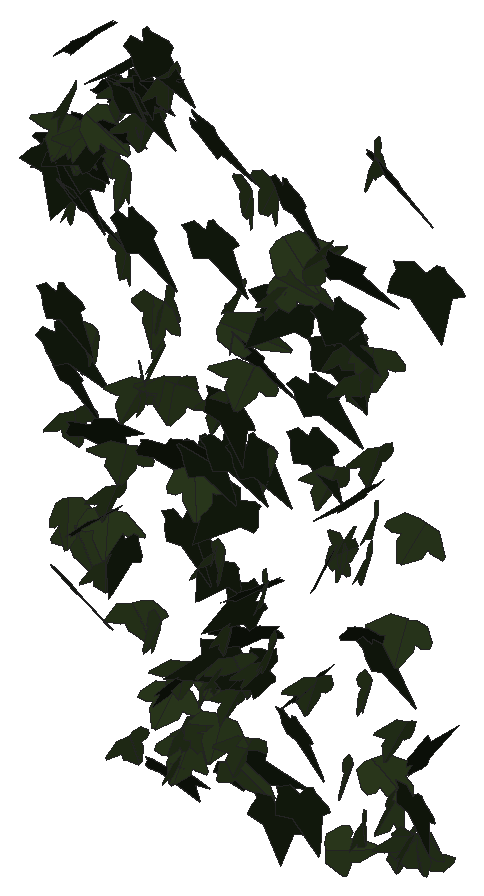
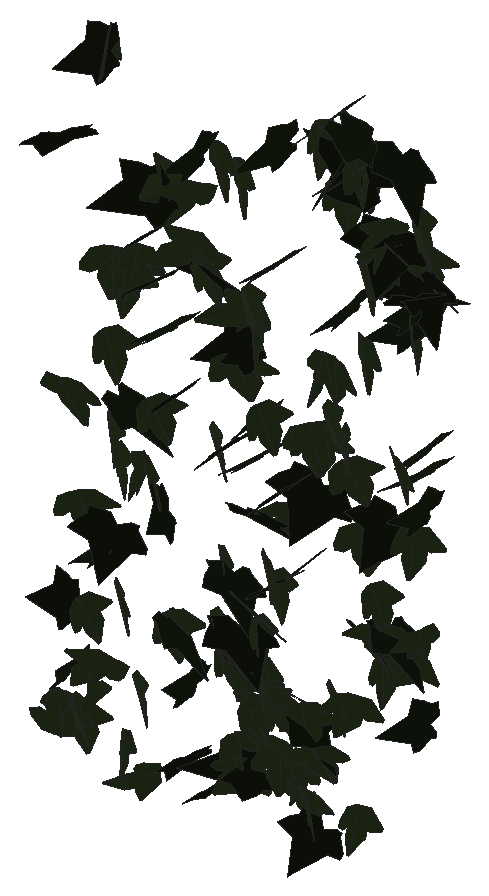
# SketchUp Ruby script. Lengths in inches.
U = 1.inch
M = Sketchup.active_model
def pt(a) = Geom::Point3d.new(a.map { |v| v * U })
def face(e, loops, mat)
  f = e.add_face(loops[0].map { |a| pt(a) })
  loops[1..].each { |l| e.add_face(l.map { |a| pt(a) }).erase! }
  f.material = f.back_material = mat if mat
  f
end
# faces: each face lists its corners as indices into pts; further lists are holes
def faces(e, pts, list, mat = nil) = list.each { |f| face(e, (f[0].is_a?(Array) ? f : [f]).map { |l| l.map { |i| pts[i] } }, mat) }
# xy, xz, yz: faces in a plane at the given z, y or x. An outline is a flat list of corners, or four numbers for a rectangle; further outlines are holes
def ring(l) = l.size == 4 ? [[l[0], l[1]], [l[2], l[1]], [l[2], l[3]], [l[0], l[3]]] : l.each_slice(2).to_a
def flat(e, list, mat, &to3) = list.each { |f| face(e, (f[0].is_a?(Array) ? f : [f]).map { |l| ring(l).map { |u, v| to3.(u, v) } }, mat) }
def xy(e, z, list, mat = nil) = flat(e, list, mat) { |x, y| [x, y, z] }
def xz(e, y, list, mat = nil) = flat(e, list, mat) { |x, z| [x, y, z] }
def yz(e, x, list, mat = nil) = flat(e, list, mat) { |y, z| [x, y, z] }
def lines(e, pts, list) = list.each { |a, b| e.add_line(pt(pts[a]), pt(pts[b])) }
# prism: a flat outline (further loops are holes) pulled along v
def prism(e, loops, v, mat = nil)
  f = face(e, loops, mat); d = Geom::Vector3d.new(v.map { |x| x * U })
  f.pushpull(f.normal.samedirection?(d) ? d.length : -d.length)
end
def box(e, o, s, mat = nil) = prism(e, [[o, [o[0] + s[0], o[1], o[2]], [o[0] + s[0], o[1] + s[1], o[2]], [o[0], o[1] + s[1], o[2]]]], [0, 0, s[2]], mat)
def at(x, y, z, deg = 0) = Geom::Transformation.translation(pt([x, y, z])) * Geom::Transformation.rotation(ORIGIN, Z_AXIS, deg.degrees)
def axes(o, x, y, z) = Geom::Transformation.new([*x, 0, *y, 0, *z, 0, *pt(o).to_a, 1])
def part(name) = M.definitions.add(name)
# library, detail: a bought-in or finely detailed component or shape, given as its bounding box
def library(name, o, s) = part(name).tap { |d| box(d.entities, o, s) }
def detail(e, o, s) = box(e.add_group.entities, o, s)
def put(e, d, t, mat = nil) = e.add_instance(d, t).tap { |i| i.material = mat if mat }
def group(e, t, mat = nil) = e.add_group.tap { |g| g.transformation = t; g.material = mat if mat }.entities
root = M.entities
M.materials.add("1026 AP 7946 SUNNY SIDE UP").color = [254, 231, 186]
M.materials.add("efeu1").color = [18, 25, 13]
M.materials.add("efeu2").color = [43, 57, 29]
c1 = part("ivyleaf_9")
p = [[1.54,2.16,1.25],[1.36,2.04,1.19],[-0.21,0.99,0.68],[-0.71,1.11,0.82],[-0.85,0.86,0.67],[-0.8,0.17,0.21],
  [-0.9,-0.01,0.1],[-0.67,-0.16,-0.02],[-0.08,-0.08,-0.05],[-0.03,-0.6,-0.4],[0.65,-0.88,-0.66],[0.83,-0.6,-0.49],
  [1.29,-0.42,-0.43],[1.8125,-0.07,-0.26],[1.21,0.44,0.15]]
faces(c1.entities,p,[[0,1,2,3,4,5,6,7,8,9,10,11,12,13,14]],"efeu1")
c2 = part("ivyleaf_10")
p = [[0,0.5,-0.03],[-0.0625,2.02,-0.43],[-0.19,2.01,-0.46],[-0.54,1.05,-0.29],[-0.52,0.625,-0.18],[-0.83,0.76,-0.28],
  [-1.16,0.64,-0.33],[-1.15,0.33,-0.24],[-0.77,-0.39,0.02],[-0.3,-0.51,0.16],[0.04,-0.48,0.23],[-0.02,2.01,-0.4375],
  [-0.06,2.01,-0.43],[0.04,-0.49,0.23],[0.67,-0.49,0.14],[1.38,0.36,-0.2],[1.375,0.51,-0.24],[0.81,0.65,-0.19],
  [0.62,0.59,-0.15],[0.6,1.09,-0.28],[0.5,1.23,-0.31]]
faces(c2.entities,p,[[0,1,2,3,4,5,6,7,8,9,10],[11,12,0,13,14,15,16,17,18,19,20]],"efeu2")
put(root,c1,axes([106.4,212.93,277.375],[0.2839,0.0766,-0.23567],[-0.3054,-0.12423,-0.20113],[-0.22609,0.264,-0.02425]),"1026 AP 7946 SUNNY SIDE UP")
put(root,c1,axes([106.09,213.01,274.86],[0.17298,-0.2627,-0.04258],[-0.00188,0.04263,-0.29273],[0.41779,0.10896,0.01631]),"1026 AP 7946 SUNNY SIDE UP")
put(root,c2,axes([106.47,212.88,277.74],[-0.41886,-0.09591,0.10877],[-0.09337,-0.12993,-0.27529],[0.20462,-0.25562,0.09702]),"1026 AP 7946 SUNNY SIDE UP")
put(root,c1,axes([106.36,212.98,277.13],[-0.301,-0.22812,-0.01885],[0.0526,-0.00599,-0.30532],[0.35582,-0.19209,0.02919]),"1026 AP 7946 SUNNY SIDE UP")
put(root,c2,axes([106.41,212.86,278.23],[0.10324,-0.30101,-0.0027],[0.009,0.00218,-0.31732],[0.47323,0.06563,0.00662]),"1026 AP 7946 SUNNY SIDE UP")
put(root,c2,axes([106.43,212.95,276.625],[0.10557,-0.27977,-0.07671],[0.01457,0.07686,-0.29473],[0.45436,0.06254,0.02728]),"1026 AP 7946 SUNNY SIDE UP")
put(root,c1,axes([106.18,212.98,273.81],[0.24349,-0.23616,0.02494],[0.02197,-0.02139,-0.29105],[0.37285,0.15548,0.00086]),"1026 AP 7946 SUNNY SIDE UP")
put(root,c1,axes([106.1875,212.96,270.41],[0.33257,-0.16333,0.03171],[0.0441,-0.01556,-0.27534],[0.25787,0.2133,0.00618]),"1026 AP 7946 SUNNY SIDE UP")
put(root,c2,axes([106.46,212.79,271.65],[0.13349,0.26405,-0.0414],[-0.0605,-0.03121,-0.28458],[-0.41595,0.08928,0.02811]),"1026 AP 7946 SUNNY SIDE UP")
put(root,c1,axes([106.25,212.8,274.36],[0.22668,-0.22817,-0.09832],[0.03052,0.11916,-0.26622],[0.38691,0.12427,0.0786]),"1026 AP 7946 SUNNY SIDE UP")
put(root,c1,axes([106.64,212.94,279.24],[-0.00906,0.30791,-0.01019],[0.00025,-0.01164,-0.31733],[-0.4845,-0.00576,0.00003]),"1026 AP 7946 SUNNY SIDE UP")
put(root,c1,axes([106.78,212.89,277.62],[-0.42856,0.13326,-0.00751],[-0.00462,-0.02428,-0.31178],[-0.20987,-0.27159,0.02221]),"1026 AP 7946 SUNNY SIDE UP")
put(root,c1,axes([106.3,212.99,276.97],[0.21519,-0.26095,0.03754],[0.01848,-0.03665,-0.3037],[0.41422,0.1372,-0.00595]),"1026 AP 7946 SUNNY SIDE UP")
put(root,c2,axes([106.56,212.79,273.18],[-0.18449,-0.25198,-0.06214],[0.05598,0.04833,-0.28582],[0.40303,-0.12206,0.01125]),"1026 AP 7946 SUNNY SIDE UP")
put(root,c1,axes([106.37,212.95,276.6875],[0.3311,-0.20967,0.01469],[0.04497,0.0069,-0.305],[0.3275,0.21102,0.02702]),"1026 AP 7946 SUNNY SIDE UP")
put(root,c2,axes([106.75,212.9375,277.65],[-0.2452,-0.23978,0.09506],[-0.01978,-0.10224,-0.29192],[0.40428,-0.15044,0.04337]),"1026 AP 7946 SUNNY SIDE UP")
put(root,c2,axes([106.62,212.85,271.26],[-0.41291,-0.03751,-0.08835],[0.14606,-0.07797,-0.25898],[0.01547,-0.26495,0.087]),"1026 AP 7946 SUNNY SIDE UP")
put(root,c2,axes([106.6875,212.99,274.39],[0.29951,-0.21338,0.00264],[0.02536,0.00935,-0.29401],[0.33462,0.19028,0.01992]),"1026 AP 7946 SUNNY SIDE UP")
put(root,c1,axes([106.91,212.84,271.62],[-0.09208,0.26235,-0.08078],[-0.00605,-0.08248,-0.27658],[-0.43119,-0.05487,0.02113]),"1026 AP 7946 SUNNY SIDE UP")
put(root,c1,axes([106.84,212.92,277.91],[0.38313,0.13865,-0.12038],[-0.17923,-0.03679,-0.28809],[-0.22276,0.26806,0.02475]),"1026 AP 7946 SUNNY SIDE UP")
put(root,c2,axes([106.78,212.91,277.55],[0.23921,0.21136,0.16111],[0.01306,0.17544,-0.25352],[-0.4121,0.12825,0.08548]),"1026 AP 7946 SUNNY SIDE UP")
put(root,c2,axes([106.9,212.85,277.98],[0.0802,0.24049,0.1869],[0.07381,0.17401,-0.25211],[-0.46659,0.06886,-0.00776]),"1026 AP 7946 SUNNY SIDE UP")
put(root,c2,axes([107.07,212.8125,270.95],[-0.07891,-0.26024,-0.07105],[0.03766,0.06406,-0.27243],[0.42107,-0.0545,0.01105]),"1026 AP 7946 SUNNY SIDE UP")
put(root,c2,axes([107.01,212.97,271.6],[0.35958,0.15229,-0.01541],[-0.01319,-0.01593,-0.283],[-0.24039,0.22868,-0.00751]),"1026 AP 7946 SUNNY SIDE UP")
put(root,c1,axes([106.98,212.66,273.22],[0.35712,0.16944,-0.00338],[0.01265,-0.01787,-0.29135],[-0.26621,0.22645,-0.01838]),"1026 AP 7946 SUNNY SIDE UP")
put(root,c2,axes([107.13,212.93,272.125],[-0.07194,-0.2743,0.01335],[-0.00541,-0.01414,-0.28657],[0.43189,-0.04587,-0.00136]),"1026 AP 7946 SUNNY SIDE UP")
put(root,c2,axes([107.3,212.94,276],[0.30258,-0.20105,-0.10219],[-0.0116,0.12357,-0.27521],[0.35154,0.17713,0.07888]),"1026 AP 7946 SUNNY SIDE UP")
put(root,c2,axes([107.28,212.97,277.23],[0.31552,-0.22148,-0.01479],[0.02757,0.03344,-0.30552],[0.34778,0.19829,0.03764]),"1026 AP 7946 SUNNY SIDE UP")
put(root,c1,axes([107.32,212.93,271.37],[-0.3046,-0.02442,-0.19731],[0.30133,-0.05585,-0.19281],[-0.03523,-0.26653,0.05684]),"1026 AP 7946 SUNNY SIDE UP")
put(root,c2,axes([107.46,212.8125,272.92],[-0.34032,-0.17094,0.04023],[-0.02467,-0.04444,-0.28322],[0.27495,-0.21557,0.02438]),"1026 AP 7946 SUNNY SIDE UP")
put(root,c2,axes([107.45,212.89,278.77],[-0.09954,-0.29918,0.04025],[0.00304,-0.04205,-0.3151],[0.47478,-0.06246,0.01046]),"1026 AP 7946 SUNNY SIDE UP")
put(root,c2,axes([107.4375,212.9,278.61],[-0.30881,0.23458,-0.03171],[0.00705,-0.03803,-0.31466],[-0.37223,-0.19533,0.02035]),"1026 AP 7946 SUNNY SIDE UP")
put(root,c1,axes([107.71,212.88,279.32],[-0.27504,0.22814,-0.12032],[0.00319,-0.14163,-0.28581],[-0.40392,-0.15646,0.07967]),"1026 AP 7946 SUNNY SIDE UP")
put(root,c2,axes([107.62,212.93,273.9375],[-0.19177,-0.22931,0.11663],[-0.02601,-0.11951,-0.26539],[0.40219,-0.11706,0.03845]),"1026 AP 7946 SUNNY SIDE UP")
put(root,c2,axes([107.5,213,270.3],[-0.29301,-0.17873,-0.06969],[0.14189,-0.00053,-0.25851],[0.26425,-0.1979,0.06153]),"1026 AP 7946 SUNNY SIDE UP")
put(root,c1,axes([107.26,212.84,278.56],[0.35939,0.19095,-0.07645],[0.07065,0.06342,0.30655],[0.31493,-0.23214,0.01848]),"1026 AP 7946 SUNNY SIDE UP")
put(root,c2,axes([107.6,212.73,268.37],[-0.1189,-0.23218,-0.1121],[0.06796,0.09889,-0.25078],[0.39652,-0.08657,0.00937]),"1026 AP 7946 SUNNY SIDE UP")
put(root,c1,axes([107.45,212.9,278.77],[0.20611,-0.26557,-0.09076],[-0.00144,0.09524,-0.3018],[0.43922,0.12494,0.0416]),"1026 AP 7946 SUNNY SIDE UP")
put(root,c2,axes([107.75,212.875,278.34],[-0.16383,-0.28736,-0.01463],[0.00738,0.01167,-0.31482],[0.45222,-0.10429,-0.00016]),"1026 AP 7946 SUNNY SIDE UP")
put(root,c1,axes([107.64,212.9,278.96],[0.27409,-0.10564,-0.23797],[-0.26091,0.16381,-0.20575],[0.30127,0.23798,0.03831]),"1026 AP 7946 SUNNY SIDE UP")
put(root,c1,axes([107.51,212.86,276.58],[0.25542,-0.26505,-0.08702],[-0.04041,0.08136,-0.31912],[0.43483,0.16325,0.02146]),"1026 AP 7946 SUNNY SIDE UP")
put(root,c2,axes([107.93,212.6,274.14],[0.02827,-0.0692,-0.30145],[-0.12562,0.2811,-0.07199],[0.45519,0.08187,-0.00115]),"1026 AP 7946 SUNNY SIDE UP")
put(root,c2,axes([107.93,212.87,270.25],[0.21508,-0.22119,-0.06482],[-0.03787,0.05756,-0.2674],[0.35907,0.13856,0.01062]),"1026 AP 7946 SUNNY SIDE UP")
put(root,c2,axes([107.99,212.82,275.41],[-0.4276,0.12187,-0.00824],[-0.05427,-0.09696,-0.28881],[-0.18429,-0.25422,0.10416]),"1026 AP 7946 SUNNY SIDE UP")
put(root,c2,axes([107.97,212.89,274.64],[0.15136,-0.27328,0.02273],[-0.00016,-0.02506,-0.2985],[0.4313,0.09589,-0.00809]),"1026 AP 7946 SUNNY SIDE UP")
put(root,c1,axes([107.79,212.84,279.54],[0.23016,-0.23822,-0.14277],[-0.04571,0.14119,-0.28361],[0.42987,0.14256,0.04628]),"1026 AP 7946 SUNNY SIDE UP")
put(root,c2,axes([108.08,212.92,275.45],[0.0443,-0.22424,-0.19395],[0.0703,0.18896,-0.2254],[0.45369,-0.00738,0.05386]),"1026 AP 7946 SUNNY SIDE UP")
put(root,c2,axes([108.12,212.89,279.11],[-0.03866,-0.29886,-0.07929],[0.0514,0.07255,-0.30735],[0.48187,-0.03172,0.02643]),"1026 AP 7946 SUNNY SIDE UP")
put(root,c2,axes([108.19,212.92,269.23],[0.34422,0.12339,-0.08412],[-0.10086,-0.05365,-0.25876],[-0.21033,0.22766,-0.01359]),"1026 AP 7946 SUNNY SIDE UP")
put(root,c1,axes([108.12,212.91,268.03],[0.38313,0.06312,-0.06072],[-0.09492,-0.00316,-0.25904],[-0.09764,0.25075,0.01358]),"1026 AP 7946 SUNNY SIDE UP")
put(root,c2,axes([108.29,212.89,274.26],[-0.21898,-0.24807,0.04203],[-0.01189,-0.04409,-0.29294],[0.39549,-0.13868,0.01446]),"1026 AP 7946 SUNNY SIDE UP")
put(root,c2,axes([108.32,212.8125,274.1875],[-0.40962,-0.10587,0.04355],[-0.04003,-0.05028,-0.28752],[0.17508,-0.25918,0.03616]),"1026 AP 7946 SUNNY SIDE UP")
put(root,c1,axes([108.46,212.8,269.62],[-0.10404,0.23036,-0.11696],[0.04624,-0.11103,-0.24755],[-0.40208,-0.07237,0.00179]),"1026 AP 7946 SUNNY SIDE UP")
put(root,c2,axes([108.39,212.79,268.29],[0.07434,-0.25314,-0.07642],[-0.00894,0.07291,-0.26475],[0.41405,0.04702,0.008]),"1026 AP 7946 SUNNY SIDE UP")
put(root,c1,axes([108.28,212.71,273.33],[0.3762,0.18498,-0.03985],[-0.02647,-0.04299,-0.31086],[-0.29631,0.23869,-0.02283]),"1026 AP 7946 SUNNY SIDE UP")
put(root,c2,axes([108.45,212.89,269.76],[-0.25281,-0.21091,0.0224],[0.0022,-0.02984,-0.27268],[0.33359,-0.15964,0.01877]),"1026 AP 7946 SUNNY SIDE UP")
put(root,c2,axes([108.47,212.85,268.46],[0.40055,-0.05555,-0.01068],[-0.01882,-0.00774,-0.26844],[0.08674,0.25482,-0.00892]),"1026 AP 7946 SUNNY SIDE UP")
put(root,c2,axes([108.54,212.74,268.82],[-0.0236,-0.21341,-0.16154],[0.07498,0.15109,-0.21735],[0.40846,-0.04006,0.03056]),"1026 AP 7946 SUNNY SIDE UP")
put(root,c1,axes([108.45,212.87,272.1],[0.12047,-0.26926,-0.02969],[-0.00909,0.02673,-0.28824],[0.42546,0.07681,0.00225]),"1026 AP 7946 SUNNY SIDE UP")
put(root,c2,axes([108.69,212.81,272.91],[0.29415,0.20877,-0.01523],[0.01552,-0.03018,-0.28758],[-0.32887,0.18531,-0.02719]),"1026 AP 7946 SUNNY SIDE UP")
put(root,c2,axes([108.89,212.84,268.9],[-0.32717,-0.16677,-0.00499],[0.02267,-0.01177,-0.27413],[0.26131,-0.20777,0.01753]),"1026 AP 7946 SUNNY SIDE UP")
put(root,c1,axes([108.66,212.97,273.3125],[0.15421,-0.24225,-0.11092],[-0.01212,0.11069,-0.26659],[0.41579,0.09307,0.03337]),"1026 AP 7946 SUNNY SIDE UP")
put(root,c2,axes([108.92,212.87,271.68],[0.01974,-0.27431,-0.03509],[0.01698,0.033,-0.28242],[0.43402,0.01119,0.01265]),"1026 AP 7946 SUNNY SIDE UP")
put(root,c2,axes([108.92,213,269.81],[0.02669,-0.23106,0.12778],[0.03711,-0.12376,-0.23904],[0.41167,0.02614,0.01326]),"1026 AP 7946 SUNNY SIDE UP")
put(root,c1,axes([109.26,212.91,270.1],[-0.40304,0.07539,0.03802],[-0.087,-0.06427,-0.26407],[-0.09885,-0.2508,0.07741]),"1026 AP 7946 SUNNY SIDE UP")
put(root,c1,axes([108.8,212.96,276.83],[0.15665,-0.27336,-0.06078],[0.02732,0.06694,-0.29671],[0.43837,0.09351,0.04021]),"1026 AP 7946 SUNNY SIDE UP")
put(root,c1,axes([109.01,213,271.61],[-0.15873,-0.21045,0.14249],[-0.04067,-0.14083,-0.23897],[0.39493,-0.09909,0.03266]),"1026 AP 7946 SUNNY SIDE UP")
put(root,c1,axes([108.84,212.77,278.64],[0.37602,-0.17227,-0.08054],[-0.05736,0.08008,-0.30002],[0.29124,0.23819,0.0449]),"1026 AP 7946 SUNNY SIDE UP")
put(root,c2,axes([109.13,212.96,274.29],[-0.09589,-0.27324,0.05986],[-0.00111,-0.06091,-0.28849],[0.43976,-0.05973,0.01233]),"1026 AP 7946 SUNNY SIDE UP")
put(root,c2,axes([109.15,212.85,269.99],[0.03642,-0.26649,-0.05086],[-0.00674,0.04766,-0.27529],[0.42568,0.02356,-0.00001]),"1026 AP 7946 SUNNY SIDE UP")
put(root,c2,axes([108.9,212.86,269.67],[0.18582,0.04657,-0.24182],[0.29934,0.14081,0.1282],[0.22867,-0.22217,0.02868]),"1026 AP 7946 SUNNY SIDE UP")
put(root,c2,axes([109.17,212.78,271.84],[0.22732,-0.22771,-0.07956],[-0.02012,0.0812,-0.2755],[0.3769,0.14168,0.03327]),"1026 AP 7946 SUNNY SIDE UP")
put(root,c2,axes([109.1,212.84,269.09],[0.42219,-0.01193,0.00195],[0.00163,-0.02067,-0.27619],[0.01894,0.26771,-0.01966]),"1026 AP 7946 SUNNY SIDE UP")
put(root,c1,axes([109.33,212.97,272.7],[-0.41821,-0.07531,-0.02714],[0.06054,-0.04249,-0.2801],[0.10963,-0.26383,0.05115]),"1026 AP 7946 SUNNY SIDE UP")
put(root,c2,axes([109.28,213.01,269.6],[-0.05165,-0.24623,0.08698],[0.00108,-0.08659,-0.25614],[0.41001,-0.03079,0.01163]),"1026 AP 7946 SUNNY SIDE UP")
put(root,c2,axes([109.26,212.93,275.57],[0.20096,-0.22477,-0.14312],[-0.0108,0.15009,-0.25817],[0.41429,0.11294,0.06269]),"1026 AP 7946 SUNNY SIDE UP")
put(root,c2,axes([109.33,212.78,270.77],[0.02695,-0.26718,-0.04215],[0.0142,0.04002,-0.27532],[0.42442,0.01563,0.01189]),"1026 AP 7946 SUNNY SIDE UP")
put(root,c2,axes([109.35,212.97,276.05],[0.10721,-0.28476,0.02012],[-0.0005,-0.02182,-0.30173],[0.44899,0.06797,-0.00514]),"1026 AP 7946 SUNNY SIDE UP")
put(root,c1,axes([109.1875,212.96,274.2],[0.04848,-0.27859,0.05016],[0.00536,-0.0502,-0.28904],[0.4451,0.03095,-0.00198]),"1026 AP 7946 SUNNY SIDE UP")
put(root,c1,axes([109.18,212.875,273.6],[0.1631,-0.25544,-0.07183],[0.04061,0.08277,-0.27815],[0.41377,0.09257,0.05561]),"1026 AP 7946 SUNNY SIDE UP")
put(root,c1,axes([109.54,212.92,270.74],[0.1217,0.23646,-0.11232],[-0.10712,-0.09282,-0.25462],[-0.39609,0.09775,0.03435]),"1026 AP 7946 SUNNY SIDE UP")
put(root,c2,axes([109.41,212.84,270.2],[-0.2553,-0.20401,-0.07447],[0.09618,0.04192,-0.26749],[0.32582,-0.17223,0.02061]),"1026 AP 7946 SUNNY SIDE UP")
put(root,c1,axes([109.66,212.9,271.24],[-0.39356,0.09785,-0.05205],[0.05519,-0.04946,-0.27509],[-0.16455,-0.25062,0.03222]),"1026 AP 7946 SUNNY SIDE UP")
put(root,c2,axes([109.58,212.89,268.91],[-0.20769,-0.21199,0.07344],[-0.02911,-0.07354,-0.25672],[0.35108,-0.1315,0.02216]),"1026 AP 7946 SUNNY SIDE UP")
put(root,c2,axes([109.64,212.88,274.9],[-0.37326,-0.14055,0.09271],[-0.03879,-0.12647,-0.26887],[0.26022,-0.22045,0.09291]),"1026 AP 7946 SUNNY SIDE UP")
put(root,c1,axes([109.72,212.83,271.49],[0.02573,0.27247,-0.01905],[-0.03757,-0.01857,-0.28033],[-0.42794,0.01801,0.02347]),"1026 AP 7946 SUNNY SIDE UP")
put(root,c2,axes([109.46,212.89,268.52],[-0.30533,-0.10503,-0.14974],[0.22815,0.03242,-0.22454],[0.16442,-0.24002,0.0335]),"1026 AP 7946 SUNNY SIDE UP")
put(root,c2,axes([109.71,212.71,277.87],[0.27223,-0.19507,-0.16176],[-0.05433,0.16918,-0.2566],[0.38888,0.16019,0.07739]),"1026 AP 7946 SUNNY SIDE UP")
put(root,c1,axes([109.39,212.87,268.57],[0.08484,0.05146,-0.26156],[0.22122,0.2123,0.07628],[0.34258,-0.14984,0.01551]),"1026 AP 7946 SUNNY SIDE UP")
put(root,c1,axes([109.39,212.87,275.31],[0.41646,-0.10912,0.05739],[0.06536,-0.04634,-0.29411],[0.18169,0.26678,-0.02575]),"1026 AP 7946 SUNNY SIDE UP")
put(root,c1,axes([109.9375,212.86,270.24],[-0.34238,0.15927,0.0061],[-0.02278,-0.01133,-0.27739],[-0.24953,-0.21751,0.01696]),"1026 AP 7946 SUNNY SIDE UP")
put(root,c2,axes([109.79,212.87,270.24],[-0.0812,-0.26715,0.02159],[-0.00896,-0.02178,-0.28043],[0.42145,-0.05193,-0.00181]),"1026 AP 7946 SUNNY SIDE UP")
put(root,c2,axes([109.5,212.7,275.64],[0.12225,0.03723,0.29408],[0.31901,0.20239,-0.08299],[-0.32069,0.21553,0.02955]),"1026 AP 7946 SUNNY SIDE UP")
put(root,c1,axes([109.63,212.86,273.7],[0.16912,-0.23692,-0.12853],[-0.02449,0.12725,-0.2649],[0.41933,0.10298,0.03636]),"1026 AP 7946 SUNNY SIDE UP")
put(root,c2,axes([109.98,212.75,271.66],[0.11497,-0.23494,-0.13312],[-0.02248,0.12896,-0.25173],[0.42001,0.07121,0.02297]),"1026 AP 7946 SUNNY SIDE UP")
put(root,c2,axes([110.01,212.86,270.66],[0.10798,-0.2627,-0.04819],[-0.00624,0.04575,-0.27935],[0.41912,0.06837,0.00826]),"1026 AP 7946 SUNNY SIDE UP")
put(root,c2,axes([110,212.88,273.59],[0.20497,-0.25546,-0.02418],[0.00378,0.02592,-0.29496],[0.40317,0.12964,0.01506]),"1026 AP 7946 SUNNY SIDE UP")
put(root,c2,axes([110.07,212.75,278.05],[0.31345,-0.18953,-0.14143],[-0.0691,0.14545,-0.27389],[0.36043,0.1927,0.07049]),"1026 AP 7946 SUNNY SIDE UP")
put(root,c2,axes([110.15,212.96,276.33],[-0.01944,-0.28822,0.05771],[-0.00416,-0.05759,-0.29753],[0.46216,-0.01264,-0.00025]),"1026 AP 7946 SUNNY SIDE UP")
put(root,c1,axes([110.08,212.9375,268.02],[-0.03618,-0.25523,0.03537],[0.00021,-0.03594,-0.26419],[0.40524,-0.02277,0.0033]),"1026 AP 7946 SUNNY SIDE UP")
put(root,c1,axes([110.36,212.96,276.22],[-0.45788,-0.02607,-0.0416],[0.06638,-0.02204,-0.30017],[0.03573,-0.29313,0.02453]),"1026 AP 7946 SUNNY SIDE UP")
put(root,c1,axes([110.22,212.9375,278.04],[0.25777,-0.25551,0.0038],[-0.01742,-0.01321,-0.31236],[0.40146,0.16348,-0.01599]),"1026 AP 7946 SUNNY SIDE UP")
put(root,c2,axes([110.27,212.92,276.53],[0.19351,0.08755,0.26416],[0.23879,0.2103,-0.14812],[-0.35194,0.19083,0.04475]),"1026 AP 7946 SUNNY SIDE UP")
put(root,c1,axes([110.38,212.89,269.55],[0.19453,-0.23128,0.05869],[0.02657,-0.05699,-0.27027],[0.3741,0.12431,-0.01132]),"1026 AP 7946 SUNNY SIDE UP")
put(root,c1,axes([110.49,212.94,268.37],[0.01379,-0.25276,-0.06532],[-0.00254,0.06195,-0.26018],[0.4092,0.0089,0.00058]),"1026 AP 7946 SUNNY SIDE UP")
put(root,c2,axes([110.51,212.71,277.28],[0.18715,0.27213,0.12238],[0.09401,0.1017,-0.3051],[-0.45634,0.13255,-0.01266]),"1026 AP 7946 SUNNY SIDE UP")
put(root,c1,axes([110.82,212.86,270.38],[-0.1959,0.22662,-0.0888],[0.04959,-0.08239,-0.26664],[-0.37874,-0.12801,0.01102]),"1026 AP 7946 SUNNY SIDE UP")
put(root,c2,axes([110.82,212.83,270.36],[-0.16025,-0.25407,0.02096],[0.00036,-0.02355,-0.282],[0.40097,-0.10152,0.00863]),"1026 AP 7946 SUNNY SIDE UP")
put(root,c1,axes([110.61,213,274.13],[0.11816,-0.2638,-0.07491],[-0.01433,0.0714,-0.28195],[0.42941,0.07497,0.0112]),"1026 AP 7946 SUNNY SIDE UP")
put(root,c1,axes([110.91,212.84,272.1],[0.02579,0.12821,0.25532],[0.09833,0.23952,-0.1309],[-0.42656,0.06296,-0.01474]),"1026 AP 7946 SUNNY SIDE UP")
put(root,c2,axes([111.04,212.96,273.74],[-0.14078,-0.25302,0.08632],[-0.00414,-0.08905,-0.27572],[0.41979,-0.08573,0.02623]),"1026 AP 7946 SUNNY SIDE UP")
put(root,c2,axes([110.97,212.64,277.18],[0.11444,-0.04208,0.32058],[-0.07772,0.31416,0.05746],[-0.48799,-0.0599,0.06603]),"1026 AP 7946 SUNNY SIDE UP")
put(root,c1,axes([110.76,212.85,275.09],[0.20512,-0.25166,-0.08618],[0.04637,0.10491,-0.28196],[0.4137,0.11302,0.07433]),"1026 AP 7946 SUNNY SIDE UP")
put(root,c2,axes([111.3,212.8,272.67],[0.19363,-0.1868,-0.17685],[-0.12981,0.14968,-0.22935],[0.37602,0.14787,0.01189]),"1026 AP 7946 SUNNY SIDE UP")
put(root,c2,axes([111.35,212.83,272.62],[-0.00527,0.08099,0.27806],[-0.18221,0.24515,-0.07596],[-0.40314,-0.11186,0.0307]),"1026 AP 7946 SUNNY SIDE UP")
put(root,c1,axes([111.07,212.99,275.75],[0.07106,-0.282,-0.06274],[0.04452,0.06408,-0.29133],[0.45093,0.03811,0.03865]),"1026 AP 7946 SUNNY SIDE UP")
put(root,c1,axes([110.98,212.92,277.16],[0.44222,-0.01893,0.10529],[0.15642,-0.03744,-0.28908],[0.04792,0.29692,-0.02797]),"1026 AP 7946 SUNNY SIDE UP")
put(root,c2,axes([111.18,212.87,267.81],[0.04604,-0.05634,-0.2737],[0.28514,0.20257,-0.02251],[0.31724,-0.17389,0.05996]),"1026 AP 7946 SUNNY SIDE UP")
put(root,c2,axes([111.39,212.86,269.16],[0.15582,-0.24641,-0.03872],[-0.0036,0.03804,-0.27311],[0.39159,0.0984,0.01289]),"1026 AP 7946 SUNNY SIDE UP")
put(root,c1,axes([111.19,212.84,276.43],[0.18087,-0.25049,-0.1249],[-0.01605,0.12578,-0.28027],[0.43631,0.10847,0.04146]),"1026 AP 7946 SUNNY SIDE UP")
put(root,c2,axes([111.42,212.82,275.96],[-0.11862,-0.25477,-0.14627],[0.07351,0.13269,-0.27287],[0.45156,-0.08852,0.006]),"1026 AP 7946 SUNNY SIDE UP")
put(root,c1,axes([111.64,212.91,273.65],[-0.23121,0.21859,-0.11049],[0.00973,-0.12328,-0.26525],[-0.38359,-0.13488,0.05987]),"1026 AP 7946 SUNNY SIDE UP")
put(root,c2,axes([111.56,212.95,268.28],[0.06004,-0.22386,-0.13155],[0.02631,0.12971,-0.23063],[0.40339,0.02486,0.03462]),"1026 AP 7946 SUNNY SIDE UP")
put(root,c2,axes([111.66,212.9375,270.57],[0.21117,-0.23207,-0.05038],[-0.01188,0.05047,-0.27527],[0.3723,0.13324,0.01979]),"1026 AP 7946 SUNNY SIDE UP")
put(root,c2,axes([111.67,212.76,275.58],[-0.15771,-0.26987,-0.07862],[0.05178,0.06752,-0.29612],[0.43729,-0.10533,0.00671]),"1026 AP 7946 SUNNY SIDE UP")
put(root,c2,axes([111.74,213.01,273.27],[0.08194,-0.24529,-0.12878],[-0.01953,0.12358,-0.25731],[0.43146,0.05218,0.01281]),"1026 AP 7946 SUNNY SIDE UP")
put(root,c2,axes([111.75,212.98,275.89],[-0.38894,-0.15536,0.00448],[0.02182,-0.03187,-0.29902],[0.24345,-0.24535,0.03396]),"1026 AP 7946 SUNNY SIDE UP")
put(root,c2,axes([111.75,212.85,272.7],[0.09567,-0.26735,-0.08169],[-0.01243,0.07792,-0.28185],[0.43764,0.06066,0.00986]),"1026 AP 7946 SUNNY SIDE UP")
put(root,c1,axes([111.79,212.875,271.55],[0.24601,0.22876,-0.02677],[-0.01257,-0.02757,-0.28553],[-0.36203,0.1564,-0.00827]),"1026 AP 7946 SUNNY SIDE UP")
put(root,c2,axes([111.9375,212.83,274.45],[-0.10321,-0.28665,0.00678],[0.00244,-0.00877,-0.30297],[0.4509,-0.06556,0.00319]),"1026 AP 7946 SUNNY SIDE UP")
put(root,c2,axes([111.97,212.74,279.21],[0.06023,-0.21093,-0.23002],[0.02668,0.22493,-0.21575],[0.48087,0.01394,0.04078]),"1026 AP 7946 SUNNY SIDE UP")
put(root,c1,axes([111.85,212.9,271.26],[0.22797,-0.23329,-0.03159],[0.00316,0.0357,-0.28197],[0.3697,0.14355,0.02189]),"1026 AP 7946 SUNNY SIDE UP")
put(root,c2,axes([111.95,212.9,269.35],[0.26189,0.16692,0.16674],[0.20121,0.09903,-0.2417],[-0.304,0.20934,-0.01633]),"1026 AP 7946 SUNNY SIDE UP")
put(root,c2,axes([112.17,212.97,268.83],[0.02056,0.11255,-0.27016],[-0.06209,-0.25993,-0.11819],[-0.44534,0.04143,0.00401]),"1026 AP 7946 SUNNY SIDE UP")
put(root,c1,axes([111.91,212.89,279.07],[0.40087,-0.17057,0.03927],[0.02596,-0.04532,-0.31492],[0.27392,0.2539,-0.02763]),"1026 AP 7946 SUNNY SIDE UP")
put(root,c2,axes([112.3,212.94,270.12],[-0.07309,-0.24965,0.08922],[-0.00496,-0.08884,-0.26182],[0.41621,-0.0449,0.01255]),"1026 AP 7946 SUNNY SIDE UP")
put(root,c2,axes([112.41,212.88,268.35],[-0.16403,-0.23957,0.02729],[-0.00208,-0.02978,-0.26913],[0.37923,-0.10378,0.01033]),"1026 AP 7946 SUNNY SIDE UP")
put(root,c2,axes([112.4,212.89,271.78],[-0.33491,-0.16326,0.07627],[0.0325,-0.13777,-0.24941],[0.28061,-0.1789,0.11992]),"1026 AP 7946 SUNNY SIDE UP")
put(root,c2,axes([112.5,212.85,268.43],[0.11016,-0.25534,0.00216],[-0.00693,-0.00488,-0.27274],[0.40147,0.06998,-0.0053]),"1026 AP 7946 SUNNY SIDE UP")
put(root,c2,axes([112.62,212.86,268.46],[-0.39556,0.05577,-0.01711],[0.01817,-0.02577,-0.26458],[-0.08982,-0.25081,0.02182]),"1026 AP 7946 SUNNY SIDE UP")
put(root,c2,axes([112.69,212.84,273.47],[0.43578,-0.04978,-0.06404],[-0.09579,0.01082,-0.29002],[0.0801,0.28376,0.00154]),"1026 AP 7946 SUNNY SIDE UP")
put(root,c1,axes([112.52,212.93,269.0625],[0.09046,-0.24616,0.07709],[0.00393,-0.07757,-0.26045],[0.40518,0.05571,-0.01468]),"1026 AP 7946 SUNNY SIDE UP")
put(root,c2,axes([112.71,212.93,268.11],[-0.32124,-0.15846,0.00052],[-0.01869,0.01762,0.26556],[-0.24847,0.20354,-0.02066]),"1026 AP 7946 SUNNY SIDE UP")
put(root,c1,axes([112.72,212.96,277.51],[-0.08523,-0.2852,-0.0761],[0.06617,0.0652,-0.29726],[0.45786,-0.06252,0.0288]),"1026 AP 7946 SUNNY SIDE UP")
put(root,c1,axes([112.8,212.625,269.89],[0.08177,0.03159,0.27598],[0.23452,0.22375,-0.05573],[-0.35309,0.15592,0.02689]),"1026 AP 7946 SUNNY SIDE UP")
